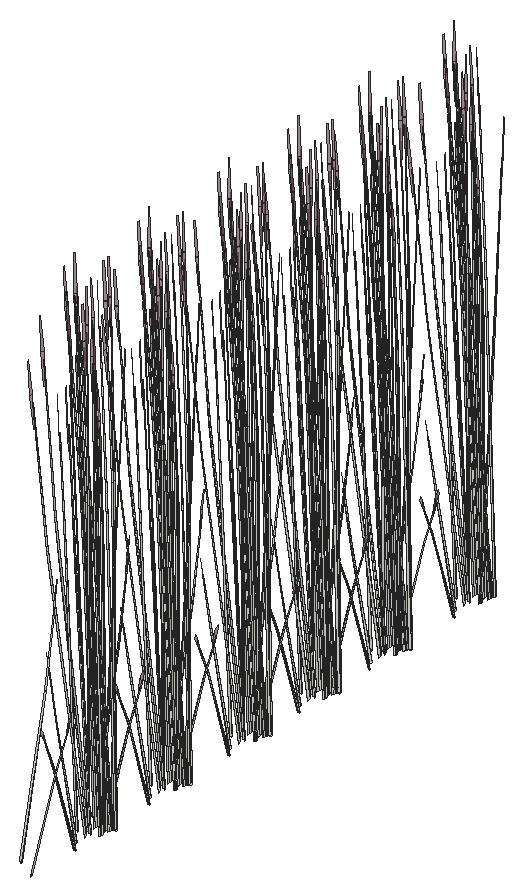
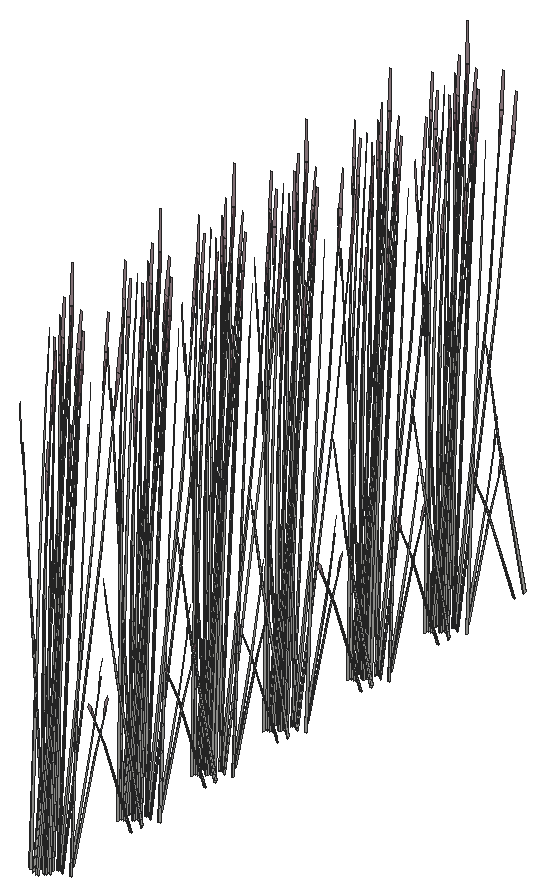
# SketchUp Ruby script. Lengths in inches.
U = 1.inch
M = Sketchup.active_model
def pt(a) = Geom::Point3d.new(a.map { |v| v * U })
def face(e, loops, mat)
  f = e.add_face(loops[0].map { |a| pt(a) })
  loops[1..].each { |l| e.add_face(l.map { |a| pt(a) }).erase! }
  f.material = f.back_material = mat if mat
  f
end
# faces: each face lists its corners as indices into pts; further lists are holes
def faces(e, pts, list, mat = nil) = list.each { |f| face(e, (f[0].is_a?(Array) ? f : [f]).map { |l| l.map { |i| pts[i] } }, mat) }
# xy, xz, yz: faces in a plane at the given z, y or x. An outline is a flat list of corners, or four numbers for a rectangle; further outlines are holes
def ring(l) = l.size == 4 ? [[l[0], l[1]], [l[2], l[1]], [l[2], l[3]], [l[0], l[3]]] : l.each_slice(2).to_a
def flat(e, list, mat, &to3) = list.each { |f| face(e, (f[0].is_a?(Array) ? f : [f]).map { |l| ring(l).map { |u, v| to3.(u, v) } }, mat) }
def xy(e, z, list, mat = nil) = flat(e, list, mat) { |x, y| [x, y, z] }
def xz(e, y, list, mat = nil) = flat(e, list, mat) { |x, z| [x, y, z] }
def yz(e, x, list, mat = nil) = flat(e, list, mat) { |y, z| [x, y, z] }
def lines(e, pts, list) = list.each { |a, b| e.add_line(pt(pts[a]), pt(pts[b])) }
# prism: a flat outline (further loops are holes) pulled along v
def prism(e, loops, v, mat = nil)
  f = face(e, loops, mat); d = Geom::Vector3d.new(v.map { |x| x * U })
  f.pushpull(f.normal.samedirection?(d) ? d.length : -d.length)
end
def box(e, o, s, mat = nil) = prism(e, [[o, [o[0] + s[0], o[1], o[2]], [o[0] + s[0], o[1] + s[1], o[2]], [o[0], o[1] + s[1], o[2]]]], [0, 0, s[2]], mat)
def at(x, y, z, deg = 0) = Geom::Transformation.translation(pt([x, y, z])) * Geom::Transformation.rotation(ORIGIN, Z_AXIS, deg.degrees)
def axes(o, x, y, z) = Geom::Transformation.new([*x, 0, *y, 0, *z, 0, *pt(o).to_a, 1])
def part(name) = M.definitions.add(name)
# library, detail: a bought-in or finely detailed component or shape, given as its bounding box
def library(name, o, s) = part(name).tap { |d| box(d.entities, o, s) }
def detail(e, o, s) = box(e.add_group.entities, o, s)
def put(e, d, t, mat = nil) = e.add_instance(d, t).tap { |i| i.material = mat if mat }
def group(e, t, mat = nil) = e.add_group.tap { |g| g.transformation = t; g.material = mat if mat }.entities
root = M.entities
M.materials.add("LightPink_Translucent").color = [144, 107, 117]
M.materials["LightPink_Translucent"].alpha = 0.75
c1 = part("blade")
p = [[2.15,0.21,22],[0,0.17,0],[0.09,0.45,0],[2.18,0.31,22],[2.29,0.31,22],[0.38,0.45,0],
  [2.48,0.24,33],[2.49,0.24,33],[2.48,0.22,33]]
faces(c1.entities,p,[[0,1,2,3],[4,5,2,3],[6,3,4,7],[8,0,3,6]])
c2 = part("seeds")
p = [[0.3,-0.1,1.38],[-0.01,-0.03,1.59],[-0.01,-0.03,0.03],[0.14,-0.07,-0.07],[0.29,-0.03,3],[0.15,0.01,3.11]]
faces(c2.entities,p,[[0,1,2,3],[1,0,4,5]],"LightPink_Translucent")
c3 = part("blade with seeds")
put(c3.entities,c1,at(0,0,0))
put(c3.entities,c2,axes([2.4,0.25,30.99],[1.5799,-0.05474,1.17369],[-0.12525,1.92788,0.29478],[-0.07173,-0.02425,1.56792]))
put(root,c3,axes([333.34,328.22,49.32],[0.08172,-0.02126,1.55816],[0.49154,0.11703,-0.23804],[0.01437,0.1319,0.26541]))
put(root,c3,axes([332.21,328.28,50.49],[0.45869,-0.0692,0.0575],[0.10545,0.27878,-0.76259],[-0.02908,0.14112,0.68355]))
put(root,c3,axes([333.7,334.08,49.32],[-0.08469,0.01408,1.55816],[-0.46834,-0.15847,-0.23804],[0.00786,-0.13218,0.26541]))
put(root,c3,axes([333,335.98,49.85],[-0.20736,-0.4007,-0.61707],[0.59731,-0.14431,-0.16195],[-0.02292,-0.13569,1.36206]))
put(root,c3,axes([333.61,334.35,49.88],[-0.34892,0.22417,-0.0344],[-0.3197,-0.24551,-0.15595],[-0.02251,-0.06957,0.51438]))
put(root,c3,axes([333.32,336.08,49.95],[0.24498,-0.3521,-0.39531],[0.50902,0.16945,0.19025],[0,-0.08116,1.26923]))
put(root,c3,axes([332.02,335.93,49.79],[0.35245,-0.2438,-0.27372],[0.35245,0.2438,0.27372],[0,-0.07853,1.22797]))
put(root,c3,axes([333.25,336.375,50.36],[-0.56863,-0.18645,-0.25709],[0.2738,-0.39352,-0.44182],[-0.01787,-0.09662,1.41118]))
put(root,c3,axes([333.42,336.14,50.09],[0.21952,0.43694,0.40429],[-0.62724,0.15194,0.15865],[0.00767,-0.08029,1.40366]))
put(root,c3,axes([333.31,336.48,50.4],[-0.24498,0.3521,0.39531],[-0.50902,-0.16945,-0.19025],[0,-0.08116,1.26923]))
put(root,c3,axes([334.36,336.52,50.03],[-0.46965,-0.33633,-0.05417],[0.46994,-0.33653,0],[-0.0164,-0.01174,1.55135]))
put(root,c3,axes([333.47,336.57,50.09],[0.63817,0.08233,0.40429],[-0.12987,0.46497,0.15865],[-0.09326,-0.0449,1.40366]))
put(root,c3,axes([333.13,337.31,50.1875],[0.54257,-0.10371,0.15589],[0.13397,0.38597,0.31002],[-0.04839,-0.05624,1.41735]))
put(root,c3,axes([333.94,337.22,49.95],[-0.16474,-0.33688,0],[0.47043,-0.11798,0],[0,0,1.36402]))
put(root,c3,axes([334.74,337.33,50.1875],[0.14586,-0.38834,0.15589],[0.53375,0.1099,0.31002],[-0.0922,0.00189,1.41735]))
put(root,c3,axes([333.83,337.37,49.94],[-0.50902,-0.17543,0],[0.24498,-0.36452,0],[0,0,1.43768]))
put(root,c3,axes([334.49,336.64,50.4],[0.54829,-0.02412,0.39531],[0.04958,0.40041,-0.19025],[-0.09816,0.04058,1.26923]))
put(root,c3,axes([334.61,337.76,49.9375],[-0.31175,-0.39292,-0.04544],[0.52815,-0.21836,0.456],[-0.13015,0.03741,1.44584]))
put(root,c3,axes([334.5,336.8125,50.3125],[0.37303,0.23477,0.12794],[-0.31115,0.26487,-0.36534],[-0.08661,0.03581,1.11991]))
put(root,c3,axes([334.89,337.54,50.19],[0.47255,-0.19538,0.43871],[0.28245,0.35034,0],[-0.10763,0.0445,1.3917]))
put(root,c3,axes([334.46,337.71,49.79],[-0.47106,-0.09668,-0.27372],[0.11861,-0.34048,0.27372],[-0.09497,0.03926,1.22797]))
put(root,c3,axes([334.38,336.73,50.36],[0.05884,0.44587,-0.25709],[-0.6128,0.02696,-0.44182],[-0.10791,0.05939,1.41118]))
put(root,c3,axes([334.61,336.55,49.95],[-0.24498,0.3521,-0.39531],[-0.50902,-0.16945,0.19025],[0,0.08116,1.26923]))
put(root,c3,axes([334.62,337.5625,50.06],[0.63212,0.12701,0.27176],[-0.15814,0.45398,-0.32244],[-0.10462,0.05682,1.45692]))
put(root,c3,axes([335,337.81,50.1],[0.31568,0.39156,0],[-0.52815,0.21836,-0.456],[-0.12029,0.04973,1.44655]))
put(root,c3,axes([333.34,337.93,49.32],[0.08172,-0.02126,1.55816],[0.49154,0.11703,-0.23804],[0.01437,0.1319,0.26541]))
put(root,c3,axes([332.21,337.98,50.49],[0.45869,-0.0692,0.0575],[0.10545,0.27878,-0.76259],[-0.02908,0.14112,0.68355]))
put(root,c3,axes([333.7,344.02,49.32],[-0.08469,0.01408,1.55816],[-0.46834,-0.15847,-0.23804],[0.00786,-0.13218,0.26541]))
put(root,c3,axes([333,345.91,49.85],[-0.20736,-0.4007,-0.61707],[0.59731,-0.14431,-0.16195],[-0.02292,-0.13569,1.36206]))
put(root,c3,axes([333.61,344.29,49.88],[-0.34892,0.22417,-0.0344],[-0.3197,-0.24551,-0.15595],[-0.02251,-0.06957,0.51438]))
put(root,c3,axes([333.32,346.02,49.95],[0.24498,-0.3521,-0.39531],[0.50902,0.16945,0.19025],[0,-0.08116,1.26923]))
put(root,c3,axes([332.02,345.87,49.79],[0.35245,-0.2438,-0.27372],[0.35245,0.2438,0.27372],[0,-0.07853,1.22797]))
put(root,c3,axes([333.25,346.31,50.36],[-0.56863,-0.18645,-0.25709],[0.2738,-0.39352,-0.44182],[-0.01787,-0.09662,1.41118]))
put(root,c3,axes([333.42,346.07,50.09],[0.21952,0.43694,0.40429],[-0.62724,0.15194,0.15865],[0.00767,-0.08029,1.40366]))
put(root,c3,axes([333.31,346.42,50.4],[-0.24498,0.3521,0.39531],[-0.50902,-0.16945,-0.19025],[0,-0.08116,1.26923]))
put(root,c3,axes([334.36,346.46,50.03],[-0.46965,-0.33633,-0.05417],[0.46994,-0.33653,0],[-0.0164,-0.01174,1.55135]))
put(root,c3,axes([333.47,346.5,50.09],[0.63817,0.08233,0.40429],[-0.12987,0.46497,0.15865],[-0.09326,-0.0449,1.40366]))
put(root,c3,axes([333.13,347.24,50.1875],[0.54257,-0.10371,0.15589],[0.13397,0.38597,0.31002],[-0.04839,-0.05624,1.41735]))
put(root,c3,axes([333.94,347.15,49.95],[-0.16474,-0.33688,0],[0.47043,-0.11798,0],[0,0,1.36402]))
put(root,c3,axes([334.74,347.26,50.1875],[0.14586,-0.38834,0.15589],[0.53375,0.1099,0.31002],[-0.0922,0.00189,1.41735]))
put(root,c3,axes([333.83,347.3,49.94],[-0.50902,-0.17543,0],[0.24498,-0.36452,0],[0,0,1.43768]))
put(root,c3,axes([334.49,346.58,50.4],[0.54829,-0.02412,0.39531],[0.04958,0.40041,-0.19025],[-0.09816,0.04058,1.26923]))
put(root,c3,axes([334.61,347.7,49.9375],[-0.31175,-0.39292,-0.04544],[0.52815,-0.21836,0.456],[-0.13015,0.03741,1.44584]))
put(root,c3,axes([334.5,346.75,50.3125],[0.37303,0.23477,0.12794],[-0.31115,0.26487,-0.36534],[-0.08661,0.03581,1.11991]))
put(root,c3,axes([334.89,347.47,50.19],[0.47255,-0.19538,0.43871],[0.28245,0.35034,0],[-0.10763,0.0445,1.3917]))
put(root,c3,axes([334.46,347.65,49.79],[-0.47106,-0.09668,-0.27372],[0.11861,-0.34048,0.27372],[-0.09497,0.03926,1.22797]))
put(root,c3,axes([334.38,346.66,50.36],[0.05884,0.44587,-0.25709],[-0.6128,0.02696,-0.44182],[-0.10791,0.05939,1.41118]))
put(root,c3,axes([334.61,346.49,49.95],[-0.24498,0.3521,-0.39531],[-0.50902,-0.16945,0.19025],[0,0.08116,1.26923]))
put(root,c3,axes([334.62,347.5,50.06],[0.63212,0.12701,0.27176],[-0.15814,0.45398,-0.32244],[-0.10462,0.05682,1.45692]))
put(root,c3,axes([335,347.74,50.1],[0.31568,0.39156,0],[-0.52815,0.21836,-0.456],[-0.12029,0.04973,1.44655]))
put(root,c3,axes([333.34,347.86,49.32],[0.08172,-0.02126,1.55816],[0.49154,0.11703,-0.23804],[0.01437,0.1319,0.26541]))
put(root,c3,axes([332.21,347.92,50.49],[0.45869,-0.0692,0.0575],[0.10545,0.27878,-0.76259],[-0.02908,0.14112,0.68355]))
put(root,c3,axes([333.7,354.74,49.32],[-0.08469,0.01408,1.55816],[-0.46834,-0.15847,-0.23804],[0.00786,-0.13218,0.26541]))
put(root,c3,axes([333,356.64,49.85],[-0.20736,-0.4007,-0.61707],[0.59731,-0.14431,-0.16195],[-0.02292,-0.13569,1.36206]))
put(root,c3,axes([333.61,355.01,49.88],[-0.34892,0.22417,-0.0344],[-0.3197,-0.24551,-0.15595],[-0.02251,-0.06957,0.51438]))
put(root,c3,axes([333.32,356.74,49.95],[0.24498,-0.3521,-0.39531],[0.50902,0.16945,0.19025],[0,-0.08116,1.26923]))
put(root,c3,axes([332.02,356.59,49.79],[0.35245,-0.2438,-0.27372],[0.35245,0.2438,0.27372],[0,-0.07853,1.22797]))
put(root,c3,axes([333.25,357.03,50.36],[-0.56863,-0.18645,-0.25709],[0.2738,-0.39352,-0.44182],[-0.01787,-0.09662,1.41118]))
put(root,c3,axes([333.42,356.79,50.09],[0.21952,0.43694,0.40429],[-0.62724,0.15194,0.15865],[0.00767,-0.08029,1.40366]))
put(root,c3,axes([333.31,357.14,50.4],[-0.24498,0.3521,0.39531],[-0.50902,-0.16945,-0.19025],[0,-0.08116,1.26923]))
put(root,c3,axes([334.36,357.18,50.03],[-0.46965,-0.33633,-0.05417],[0.46994,-0.33653,0],[-0.0164,-0.01174,1.55135]))
put(root,c3,axes([333.47,357.22,50.09],[0.63817,0.08233,0.40429],[-0.12987,0.46497,0.15865],[-0.09326,-0.0449,1.40366]))
put(root,c3,axes([333.13,357.97,50.1875],[0.54257,-0.10371,0.15589],[0.13397,0.38597,0.31002],[-0.04839,-0.05624,1.41735]))
put(root,c3,axes([333.94,357.875,49.95],[-0.16474,-0.33688,0],[0.47043,-0.11798,0],[0,0,1.36402]))
put(root,c3,axes([334.74,357.99,50.1875],[0.14586,-0.38834,0.15589],[0.53375,0.1099,0.31002],[-0.0922,0.00189,1.41735]))
put(root,c3,axes([333.83,358.03,49.94],[-0.50902,-0.17543,0],[0.24498,-0.36452,0],[0,0,1.43768]))
put(root,c3,axes([334.49,357.3,50.4],[0.54829,-0.02412,0.39531],[0.04958,0.40041,-0.19025],[-0.09816,0.04058,1.26923]))
put(root,c3,axes([334.61,358.42,49.9375],[-0.31175,-0.39292,-0.04544],[0.52815,-0.21836,0.456],[-0.13015,0.03741,1.44584]))
put(root,c3,axes([334.5,357.47,50.3125],[0.37303,0.23477,0.12794],[-0.31115,0.26487,-0.36534],[-0.08661,0.03581,1.11991]))
put(root,c3,axes([334.89,358.2,50.19],[0.47255,-0.19538,0.43871],[0.28245,0.35034,0],[-0.10763,0.0445,1.3917]))
put(root,c3,axes([334.46,358.37,49.79],[-0.47106,-0.09668,-0.27372],[0.11861,-0.34048,0.27372],[-0.09497,0.03926,1.22797]))
put(root,c3,axes([334.38,357.39,50.36],[0.05884,0.44587,-0.25709],[-0.6128,0.02696,-0.44182],[-0.10791,0.05939,1.41118]))
put(root,c3,axes([334.61,357.21,49.95],[-0.24498,0.3521,-0.39531],[-0.50902,-0.16945,0.19025],[0,0.08116,1.26923]))
put(root,c3,axes([334.62,358.22,50.06],[0.63212,0.12701,0.27176],[-0.15814,0.45398,-0.32244],[-0.10462,0.05682,1.45692]))
put(root,c3,axes([335,358.47,50.1],[0.31568,0.39156,0],[-0.52815,0.21836,-0.456],[-0.12029,0.04973,1.44655]))
put(root,c3,axes([333.34,358.59,49.32],[0.08172,-0.02126,1.55816],[0.49154,0.11703,-0.23804],[0.01437,0.1319,0.26541]))
put(root,c3,axes([332.21,358.64,50.49],[0.45869,-0.0692,0.0575],[0.10545,0.27878,-0.76259],[-0.02908,0.14112,0.68355]))
put(root,c3,axes([333.7,364.0625,49.32],[-0.08469,0.01408,1.55816],[-0.46834,-0.15847,-0.23804],[0.00786,-0.13218,0.26541]))
put(root,c3,axes([333,365.96,49.85],[-0.20736,-0.4007,-0.61707],[0.59731,-0.14431,-0.16195],[-0.02292,-0.13569,1.36206]))
put(root,c3,axes([333.61,364.34,49.88],[-0.34892,0.22417,-0.0344],[-0.3197,-0.24551,-0.15595],[-0.02251,-0.06957,0.51438]))
put(root,c3,axes([333.32,366.07,49.95],[0.24498,-0.3521,-0.39531],[0.50902,0.16945,0.19025],[0,-0.08116,1.26923]))
put(root,c3,axes([332.02,365.91,49.79],[0.35245,-0.2438,-0.27372],[0.35245,0.2438,0.27372],[0,-0.07853,1.22797]))
put(root,c3,axes([333.25,366.36,50.36],[-0.56863,-0.18645,-0.25709],[0.2738,-0.39352,-0.44182],[-0.01787,-0.09662,1.41118]))
put(root,c3,axes([333.42,366.12,50.09],[0.21952,0.43694,0.40429],[-0.62724,0.15194,0.15865],[0.00767,-0.08029,1.40366]))
put(root,c3,axes([333.31,366.46,50.4],[-0.24498,0.3521,0.39531],[-0.50902,-0.16945,-0.19025],[0,-0.08116,1.26923]))
put(root,c3,axes([334.36,366.51,50.03],[-0.46965,-0.33633,-0.05417],[0.46994,-0.33653,0],[-0.0164,-0.01174,1.55135]))
put(root,c3,axes([333.47,366.55,50.09],[0.63817,0.08233,0.40429],[-0.12987,0.46497,0.15865],[-0.09326,-0.0449,1.40366]))
put(root,c3,axes([333.13,367.29,50.1875],[0.54257,-0.10371,0.15589],[0.13397,0.38597,0.31002],[-0.04839,-0.05624,1.41735]))
put(root,c3,axes([333.94,367.2,49.95],[-0.16474,-0.33688,0],[0.47043,-0.11798,0],[0,0,1.36402]))
put(root,c3,axes([334.74,367.3125,50.1875],[0.14586,-0.38834,0.15589],[0.53375,0.1099,0.31002],[-0.0922,0.00189,1.41735]))
put(root,c3,axes([333.83,367.35,49.94],[-0.50902,-0.17543,0],[0.24498,-0.36452,0],[0,0,1.43768]))
put(root,c3,axes([334.49,366.625,50.4],[0.54829,-0.02412,0.39531],[0.04958,0.40041,-0.19025],[-0.09816,0.04058,1.26923]))
put(root,c3,axes([334.61,367.75,49.9375],[-0.31175,-0.39292,-0.04544],[0.52815,-0.21836,0.456],[-0.13015,0.03741,1.44584]))
put(root,c3,axes([334.5,366.8,50.3125],[0.37303,0.23477,0.12794],[-0.31115,0.26487,-0.36534],[-0.08661,0.03581,1.11991]))
put(root,c3,axes([334.89,367.52,50.19],[0.47255,-0.19538,0.43871],[0.28245,0.35034,0],[-0.10763,0.0445,1.3917]))
put(root,c3,axes([334.46,367.7,49.79],[-0.47106,-0.09668,-0.27372],[0.11861,-0.34048,0.27372],[-0.09497,0.03926,1.22797]))
put(root,c3,axes([334.38,366.71,50.36],[0.05884,0.44587,-0.25709],[-0.6128,0.02696,-0.44182],[-0.10791,0.05939,1.41118]))
put(root,c3,axes([334.61,366.54,49.95],[-0.24498,0.3521,-0.39531],[-0.50902,-0.16945,0.19025],[0,0.08116,1.26923]))
put(root,c3,axes([334.62,367.55,50.06],[0.63212,0.12701,0.27176],[-0.15814,0.45398,-0.32244],[-0.10462,0.05682,1.45692]))
put(root,c3,axes([335,367.79,50.1],[0.31568,0.39156,0],[-0.52815,0.21836,-0.456],[-0.12029,0.04973,1.44655]))
put(root,c3,axes([333.34,367.91,49.32],[0.08172,-0.02126,1.55816],[0.49154,0.11703,-0.23804],[0.01437,0.1319,0.26541]))
put(root,c3,axes([332.21,367.96,50.49],[0.45869,-0.0692,0.0575],[0.10545,0.27878,-0.76259],[-0.02908,0.14112,0.68355]))
put(root,c3,axes([333.7,373.54,49.32],[-0.08469,0.01408,1.55816],[-0.46834,-0.15847,-0.23804],[0.00786,-0.13218,0.26541]))
put(root,c3,axes([333,375.43,49.85],[-0.20736,-0.4007,-0.61707],[0.59731,-0.14431,-0.16195],[-0.02292,-0.13569,1.36206]))
put(root,c3,axes([333.61,373.81,49.88],[-0.34892,0.22417,-0.0344],[-0.3197,-0.24551,-0.15595],[-0.02251,-0.06957,0.51438]))
put(root,c3,axes([333.32,375.54,49.95],[0.24498,-0.3521,-0.39531],[0.50902,0.16945,0.19025],[0,-0.08116,1.26923]))
put(root,c3,axes([332.02,375.39,49.79],[0.35245,-0.2438,-0.27372],[0.35245,0.2438,0.27372],[0,-0.07853,1.22797]))
put(root,c3,axes([333.25,375.83,50.36],[-0.56863,-0.18645,-0.25709],[0.2738,-0.39352,-0.44182],[-0.01787,-0.09662,1.41118]))
put(root,c3,axes([333.42,375.59,50.09],[0.21952,0.43694,0.40429],[-0.62724,0.15194,0.15865],[0.00767,-0.08029,1.40366]))
put(root,c3,axes([333.31,375.9375,50.4],[-0.24498,0.3521,0.39531],[-0.50902,-0.16945,-0.19025],[0,-0.08116,1.26923]))
put(root,c3,axes([334.36,375.98,50.03],[-0.46965,-0.33633,-0.05417],[0.46994,-0.33653,0],[-0.0164,-0.01174,1.55135]))
put(root,c3,axes([333.47,376.02,50.09],[0.63817,0.08233,0.40429],[-0.12987,0.46497,0.15865],[-0.09326,-0.0449,1.40366]))
put(root,c3,axes([333.13,376.76,50.1875],[0.54257,-0.10371,0.15589],[0.13397,0.38597,0.31002],[-0.04839,-0.05624,1.41735]))
put(root,c3,axes([333.94,376.67,49.95],[-0.16474,-0.33688,0],[0.47043,-0.11798,0],[0,0,1.36402]))
put(root,c3,axes([334.74,376.79,50.1875],[0.14586,-0.38834,0.15589],[0.53375,0.1099,0.31002],[-0.0922,0.00189,1.41735]))
put(root,c3,axes([333.83,376.83,49.94],[-0.50902,-0.17543,0],[0.24498,-0.36452,0],[0,0,1.43768]))
put(root,c3,axes([334.49,376.1,50.4],[0.54829,-0.02412,0.39531],[0.04958,0.40041,-0.19025],[-0.09816,0.04058,1.26923]))
put(root,c3,axes([334.61,377.22,49.9375],[-0.31175,-0.39292,-0.04544],[0.52815,-0.21836,0.456],[-0.13015,0.03741,1.44584]))
put(root,c3,axes([334.5,376.27,50.3125],[0.37303,0.23477,0.12794],[-0.31115,0.26487,-0.36534],[-0.08661,0.03581,1.11991]))
put(root,c3,axes([334.89,376.99,50.19],[0.47255,-0.19538,0.43871],[0.28245,0.35034,0],[-0.10763,0.0445,1.3917]))
put(root,c3,axes([334.46,377.17,49.79],[-0.47106,-0.09668,-0.27372],[0.11861,-0.34048,0.27372],[-0.09497,0.03926,1.22797]))
put(root,c3,axes([334.38,376.18,50.36],[0.05884,0.44587,-0.25709],[-0.6128,0.02696,-0.44182],[-0.10791,0.05939,1.41118]))
put(root,c3,axes([334.61,376.01,49.95],[-0.24498,0.3521,-0.39531],[-0.50902,-0.16945,0.19025],[0,0.08116,1.26923]))
put(root,c3,axes([334.62,377.02,50.06],[0.63212,0.12701,0.27176],[-0.15814,0.45398,-0.32244],[-0.10462,0.05682,1.45692]))
put(root,c3,axes([335,377.26,50.1],[0.31568,0.39156,0],[-0.52815,0.21836,-0.456],[-0.12029,0.04973,1.44655]))
put(root,c3,axes([333.34,377.38,49.32],[0.08172,-0.02126,1.55816],[0.49154,0.11703,-0.23804],[0.01437,0.1319,0.26541]))
put(root,c3,axes([332.21,377.4375,50.49],[0.45869,-0.0692,0.0575],[0.10545,0.27878,-0.76259],[-0.02908,0.14112,0.68355]))
put(root,c3,axes([333.7,384.84,49.32],[-0.08469,0.01408,1.55816],[-0.46834,-0.15847,-0.23804],[0.00786,-0.13218,0.26541]))
put(root,c3,axes([333,386.74,49.85],[-0.20736,-0.4007,-0.61707],[0.59731,-0.14431,-0.16195],[-0.02292,-0.13569,1.36206]))
put(root,c3,axes([333.61,385.12,49.88],[-0.34892,0.22417,-0.0344],[-0.3197,-0.24551,-0.15595],[-0.02251,-0.06957,0.51438]))
put(root,c3,axes([333.32,386.85,49.95],[0.24498,-0.3521,-0.39531],[0.50902,0.16945,0.19025],[0,-0.08116,1.26923]))
put(root,c3,axes([332.02,386.7,49.79],[0.35245,-0.2438,-0.27372],[0.35245,0.2438,0.27372],[0,-0.07853,1.22797]))
put(root,c3,axes([333.25,387.14,50.36],[-0.56863,-0.18645,-0.25709],[0.2738,-0.39352,-0.44182],[-0.01787,-0.09662,1.41118]))
put(root,c3,axes([333.42,386.9,50.09],[0.21952,0.43694,0.40429],[-0.62724,0.15194,0.15865],[0.00767,-0.08029,1.40366]))
put(root,c3,axes([333.31,387.25,50.4],[-0.24498,0.3521,0.39531],[-0.50902,-0.16945,-0.19025],[0,-0.08116,1.26923]))
put(root,c3,axes([334.36,387.29,50.03],[-0.46965,-0.33633,-0.05417],[0.46994,-0.33653,0],[-0.0164,-0.01174,1.55135]))
put(root,c3,axes([333.47,387.33,50.09],[0.63817,0.08233,0.40429],[-0.12987,0.46497,0.15865],[-0.09326,-0.0449,1.40366]))
put(root,c3,axes([333.13,388.07,50.1875],[0.54257,-0.10371,0.15589],[0.13397,0.38597,0.31002],[-0.04839,-0.05624,1.41735]))
put(root,c3,axes([333.94,387.98,49.95],[-0.16474,-0.33688,0],[0.47043,-0.11798,0],[0,0,1.36402]))
put(root,c3,axes([334.74,388.09,50.1875],[0.14586,-0.38834,0.15589],[0.53375,0.1099,0.31002],[-0.0922,0.00189,1.41735]))
put(root,c3,axes([333.83,388.13,49.94],[-0.50902,-0.17543,0],[0.24498,-0.36452,0],[0,0,1.43768]))
put(root,c3,axes([334.49,387.41,50.4],[0.54829,-0.02412,0.39531],[0.04958,0.40041,-0.19025],[-0.09816,0.04058,1.26923]))
put(root,c3,axes([334.61,388.53,49.9375],[-0.31175,-0.39292,-0.04544],[0.52815,-0.21836,0.456],[-0.13015,0.03741,1.44584]))
put(root,c3,axes([334.5,387.58,50.3125],[0.37303,0.23477,0.12794],[-0.31115,0.26487,-0.36534],[-0.08661,0.03581,1.11991]))
put(root,c3,axes([334.89,388.3,50.19],[0.47255,-0.19538,0.43871],[0.28245,0.35034,0],[-0.10763,0.0445,1.3917]))
put(root,c3,axes([334.46,388.48,49.79],[-0.47106,-0.09668,-0.27372],[0.11861,-0.34048,0.27372],[-0.09497,0.03926,1.22797]))
put(root,c3,axes([334.38,387.49,50.36],[0.05884,0.44587,-0.25709],[-0.6128,0.02696,-0.44182],[-0.10791,0.05939,1.41118]))
put(root,c3,axes([334.61,387.32,49.95],[-0.24498,0.3521,-0.39531],[-0.50902,-0.16945,0.19025],[0,0.08116,1.26923]))
